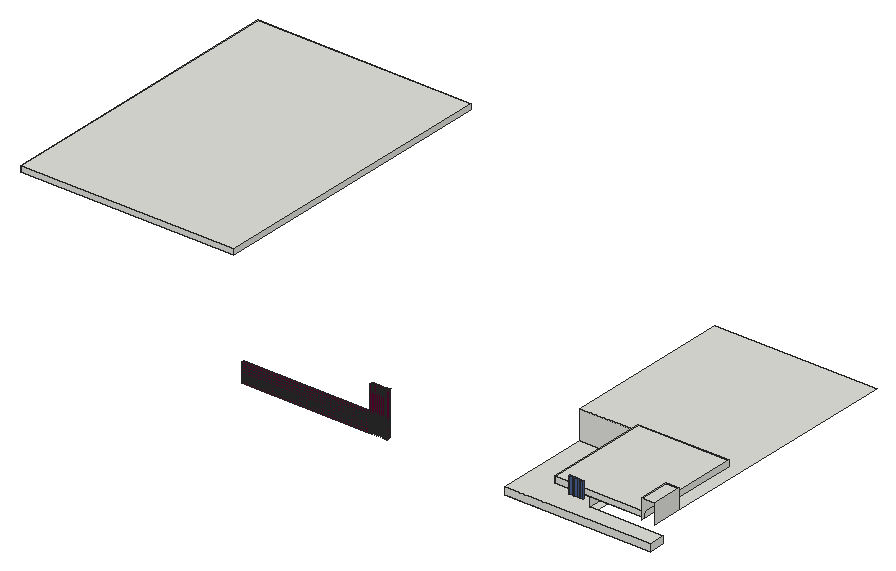
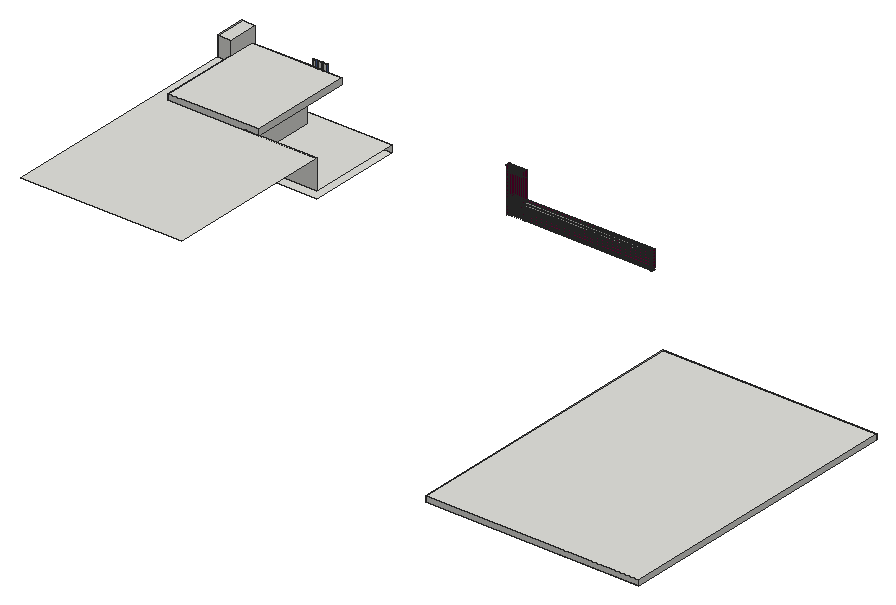
# SketchUp Ruby script. Lengths in inches.
U = 1.inch
M = Sketchup.active_model
def pt(a) = Geom::Point3d.new(a.map { |v| v * U })
def face(e, loops, mat)
  f = e.add_face(loops[0].map { |a| pt(a) })
  loops[1..].each { |l| e.add_face(l.map { |a| pt(a) }).erase! }
  f.material = f.back_material = mat if mat
  f
end
# faces: each face lists its corners as indices into pts; further lists are holes
def faces(e, pts, list, mat = nil) = list.each { |f| face(e, (f[0].is_a?(Array) ? f : [f]).map { |l| l.map { |i| pts[i] } }, mat) }
# xy, xz, yz: faces in a plane at the given z, y or x. An outline is a flat list of corners, or four numbers for a rectangle; further outlines are holes
def ring(l) = l.size == 4 ? [[l[0], l[1]], [l[2], l[1]], [l[2], l[3]], [l[0], l[3]]] : l.each_slice(2).to_a
def flat(e, list, mat, &to3) = list.each { |f| face(e, (f[0].is_a?(Array) ? f : [f]).map { |l| ring(l).map { |u, v| to3.(u, v) } }, mat) }
def xy(e, z, list, mat = nil) = flat(e, list, mat) { |x, y| [x, y, z] }
def xz(e, y, list, mat = nil) = flat(e, list, mat) { |x, z| [x, y, z] }
def yz(e, x, list, mat = nil) = flat(e, list, mat) { |y, z| [x, y, z] }
def lines(e, pts, list) = list.each { |a, b| e.add_line(pt(pts[a]), pt(pts[b])) }
# prism: a flat outline (further loops are holes) pulled along v
def prism(e, loops, v, mat = nil)
  f = face(e, loops, mat); d = Geom::Vector3d.new(v.map { |x| x * U })
  f.pushpull(f.normal.samedirection?(d) ? d.length : -d.length)
end
def box(e, o, s, mat = nil) = prism(e, [[o, [o[0] + s[0], o[1], o[2]], [o[0] + s[0], o[1] + s[1], o[2]], [o[0], o[1] + s[1], o[2]]]], [0, 0, s[2]], mat)
def at(x, y, z, deg = 0) = Geom::Transformation.translation(pt([x, y, z])) * Geom::Transformation.rotation(ORIGIN, Z_AXIS, deg.degrees)
def axes(o, x, y, z) = Geom::Transformation.new([*x, 0, *y, 0, *z, 0, *pt(o).to_a, 1])
def part(name) = M.definitions.add(name)
# library, detail: a bought-in or finely detailed component or shape, given as its bounding box
def library(name, o, s) = part(name).tap { |d| box(d.entities, o, s) }
def detail(e, o, s) = box(e.add_group.entities, o, s)
def put(e, d, t, mat = nil) = e.add_instance(d, t).tap { |i| i.material = mat if mat }
def group(e, t, mat = nil) = e.add_group.tap { |g| g.transformation = t; g.material = mat if mat }.entities
root = M.entities
M.materials.add("[Color L16]").color = [102, 0, 51]
M.materials.add("[Formica Blue]").color = [71, 97, 152]
c1 = part("Recessed downlight \#2")
detail(c1.entities,[0,0,0],[12.875,12.875,1.625])
box(root,[182.534,303.729,246],[321,447,8])
xy(root,218.208,[[671.442,109.729,862.505,112.729]],"[Color L16]")
xy(root,220.302,[[671.442,109.729,862.505,112.729]],"[Color L16]")
xy(root,222,[[1084.247,87.973,1192.934,229.266],[1192.934,87.973,1303.381,111.973]])
xy(root,222.154,[[671.442,109.729,862.505,112.729]],"[Color L16]")
xy(root,224.248,[[671.442,109.729,862.505,112.729]],"[Color L16]")
xy(root,226.101,[[671.442,109.729,862.505,112.729]],"[Color L16]")
xy(root,228.195,[[671.442,109.729,862.505,112.729]],"[Color L16]")
xy(root,230.047,[[671.442,109.729,862.505,112.729]],"[Color L16]")
xy(root,232.141,[[671.442,109.729,862.505,112.729]],"[Color L16]")
xy(root,232.677,[[1084.247,87.973,1303.381,87.973,1303.381,111.973,1192.934,111.973,1192.934,229.266,1084.247,229.266]])
xy(root,233.993,[[671.442,109.729,862.505,112.729]],"[Color L16]")
xy(root,236.087,[[671.442,109.729,862.505,112.729]],"[Color L16]")
xy(root,237.94,[[671.442,109.729,862.505,112.729]],"[Color L16]")
xy(root,240.034,[[671.442,109.729,862.505,112.729]],"[Color L16]")
xy(root,241.886,[[671.442,109.729,862.505,112.729]],"[Color L16]")
xy(root,243.98,[[671.442,109.729,862.505,112.729]],"[Color L16]")
xy(root,245.953,[[671.442,109.729,862.505,112.729]],"[Color L16]")
xy(root,269.993,[[1210.986,69.91,1216.514,71.91]])
xy(root,269.993,[[1195.298,69.91,1200.826,71.91],[1202.736,69.91,1208.264,71.91]],"[Formica Blue]")
xy(root,275.672,[[889.414,108.916,889.428,112.729],[864.033,109.729,864.088,112.729],[867.208,109.729,867.254,112.729],[868.722,109.729,868.782,112.729],[870.382,109.729,870.419,112.729],
  [871.896,109.729,871.948,112.729],[873.556,109.729,873.585,112.729],[875.071,109.729,875.113,112.729],[876.731,109.729,876.751,112.729],[878.245,109.729,878.279,112.729],
  [879.905,109.729,879.917,112.729],[881.419,109.729,881.445,112.729],[883.079,109.729,883.082,112.729],[884.594,109.729,884.611,112.729],[886.248,110.041,886.254,112.729],
  [887.768,110.041,887.831,112.729],[889.414,112.729,889.428,114.354]],"[Color L16]")
xy(root,275.806,[[1171.934,71.91,1171.934,229.266,1192.934,229.266,1192.934,111.973,1307.818,111.973,1307.818,71.91]])
xy(root,276.1875,[[1307.818,111.973,1327.309,111.973,1327.309,482.785,1084.247,482.785,1084.247,229.266,1307.818,229.266]])
xy(root,284.75,[[1171.934,71.91,1307.818,229.266]])
xy(root,284.941,[[889.428,108.916,890.942,114.354],[864.033,109.729,865.547,112.729],[867.208,109.729,868.722,112.729],[870.382,109.729,871.896,112.729],[873.556,109.729,875.071,112.729],
  [876.731,109.729,878.245,112.729],[879.905,109.729,881.419,112.729],[883.079,109.729,884.594,112.729],[886.254,110.041,887.768,112.729]],"[Color L16]")
xy(root,294,[[1210.986,69.91,1216.514,71.91]],"[Formica Blue]")
xy(root,294.25,[[1195.298,69.91,1200.826,71.91],[1202.736,69.91,1208.264,71.91]],"[Formica Blue]")
xz(root,69.91,[[1195.298,269.993,1200.826,294.25],[1202.736,269.993,1208.264,294.25],[1210.986,269.993,1216.514,294]],"[Formica Blue]")
xz(root,71.91,[[1195.298,269.993,1200.826,275.806],[1202.736,269.993,1208.264,275.806],[1210.986,269.993,1216.514,275.806],[1171.934,275.806,1195.298,284.75],[1195.298,275.806,1200.826,284.75],
  [1200.826,275.806,1202.736,284.75],[1202.736,275.806,1208.264,284.75],[1208.264,275.806,1210.986,284.75],[1210.986,275.806,1216.514,284.75],[1216.514,275.806,1307.818,275.806,1307.643,284.75,1216.514,284.75],
  [1307.818,275.806,1307.818,284.75,1307.643,284.75],[1195.298,284.75,1200.826,294.25],[1202.736,284.75,1208.264,294.25],[1210.986,284.75,1216.514,294]])
xz(root,87.973,[[1084.247,222,1303.381,232.677]])
xz(root,109.729,[[671.442,220.302,862.505,222.154],[671.442,224.248,862.505,226.101],[671.442,228.195,862.505,230.047],[671.442,232.141,862.505,233.993],[671.442,236.087,862.505,237.94],
  [671.442,240.034,862.505,241.886],[671.442,243.98,862.505,245.953]],"[Color L16]")
xz(root,111.973,[[1307.818,275.806,1307.248,304.925,1326.739,305.307,1327.309,276.1875,1307.818,276.1875],[1307.818,275.806,1307.818,276.1875,1327.309,276.1875]])
xz(root,112.729,[[671.442,218.208,862.505,218.329],[671.442,218.329,862.505,220.181],[671.442,220.181,862.505,220.302],[671.442,222.154,862.505,222.275],[671.442,222.275,862.505,224.127],
  [671.442,224.127,862.505,224.248],[671.442,226.101,862.505,226.221],[671.442,226.221,862.505,228.074],[671.442,228.074,862.505,228.195],[671.442,230.047,862.505,230.168],
  [671.442,230.168,862.505,232.02],[671.442,232.02,862.505,232.141],[671.442,233.993,862.505,234.114],[671.442,234.114,862.505,235.967],[671.442,235.967,862.505,236.087],
  [671.442,237.94,862.505,238.061],[671.442,238.061,862.505,239.913],[671.442,239.913,862.505,240.034],[671.442,241.886,862.505,242.007],[671.442,242.007,862.505,243.86],
  [671.442,243.86,862.505,243.98],[867.135,275.672,867.208,284.941],[868.722,275.672,868.795,284.941],[870.309,275.672,870.382,284.941],[871.896,275.672,871.969,284.941],
  [873.483,275.672,873.556,284.941],[875.071,275.672,875.143,284.941],[876.658,275.672,876.731,284.941],[878.245,275.672,878.318,284.941],[879.832,275.672,879.905,284.941],
  [881.419,275.672,881.492,284.941],[883.006,275.672,883.079,284.941],[884.594,275.672,884.667,284.941],[886.181,275.672,886.254,284.941]])
xz(root,112.729,[[887.768,275.672,887.841,284.941]],"[Color L16]")
xz(root,229.266,[[1084.247,232.677,1192.934,232.677,1192.934,275.806,1171.934,275.806,1171.934,276.1875,1084.247,276.1875],[1171.934,275.806,1192.934,276.1875],[1171.934,276.1875,1307.818,284.75]])
yz(root,671.442,[[109.729,220.302,112.729,222.154],[109.729,224.248,112.729,226.101],[109.729,228.195,112.729,230.047],[109.729,232.141,112.729,233.993],[109.729,236.087,112.729,237.94],
  [109.729,240.034,112.729,241.886],[109.729,243.98,112.729,245.953]],"[Color L16]")
yz(root,862.505,[[109.729,220.302,112.729,222.154],[109.729,224.248,112.729,226.101],[109.729,228.195,112.729,230.047],[109.729,232.141,112.729,233.993],[109.729,236.087,112.729,237.94],
  [109.729,240.034,112.729,241.886],[109.729,243.98,112.729,245.953]],"[Color L16]")
yz(root,864.033,[[109.729,275.672,112.729,284.941]],"[Color L16]")
yz(root,864.088,[[109.729,218.208,112.729,218.329],[109.729,218.329,112.729,220.181],[109.729,220.181,112.729,220.302],[109.729,220.302,112.729,222.154],[109.729,222.154,112.729,222.275],
  [109.729,222.275,112.729,224.127],[109.729,224.127,112.729,224.248],[109.729,224.248,112.729,226.101],[109.729,226.101,112.729,226.221],[109.729,226.221,112.729,228.074],
  [109.729,228.074,112.729,228.195],[109.729,228.195,112.729,230.047],[109.729,230.047,112.729,230.168],[109.729,230.168,112.729,232.02],[109.729,232.02,112.729,232.141],
  [109.729,232.141,112.729,233.993],[109.729,233.993,112.729,234.114],[109.729,234.114,112.729,235.967],[109.729,235.967,112.729,236.087],[109.729,236.087,112.729,237.94],
  [109.729,237.94,112.729,238.061],[109.729,238.061,112.729,239.913],[109.729,239.913,112.729,240.034],[109.729,240.034,112.729,241.886],[109.729,241.886,112.729,242.007],
  [109.729,242.007,112.729,243.86],[109.729,243.86,112.729,243.98],[109.729,243.98,112.729,245.953],[109.729,245.953,112.729,275.672]],"[Color L16]")
yz(root,867.208,[[109.729,275.672,112.729,284.941]],"[Color L16]")
yz(root,867.254,[[109.729,218.208,112.729,218.329],[109.729,218.329,112.729,220.181],[109.729,220.181,112.729,220.302],[109.729,220.302,112.729,222.154],[109.729,222.154,112.729,222.275],
  [109.729,222.275,112.729,224.127],[109.729,224.127,112.729,224.248],[109.729,224.248,112.729,226.101],[109.729,226.101,112.729,226.221],[109.729,226.221,112.729,228.074],
  [109.729,228.074,112.729,228.195],[109.729,228.195,112.729,230.047],[109.729,230.047,112.729,230.168],[109.729,230.168,112.729,232.02],[109.729,232.02,112.729,232.141],
  [109.729,232.141,112.729,233.993],[109.729,233.993,112.729,234.114],[109.729,234.114,112.729,235.967],[109.729,235.967,112.729,236.087],[109.729,236.087,112.729,237.94],
  [109.729,237.94,112.729,238.061],[109.729,238.061,112.729,239.913],[109.729,239.913,112.729,240.034],[109.729,240.034,112.729,241.886],[109.729,241.886,112.729,242.007],
  [109.729,242.007,112.729,243.86],[109.729,243.86,112.729,243.98],[109.729,243.98,112.729,245.953],[109.729,245.953,112.729,275.672]],"[Color L16]")
yz(root,868.722,[[109.729,275.672,112.729,284.941]],"[Color L16]")
yz(root,870.382,[[109.729,275.672,112.729,284.941]],"[Color L16]")
yz(root,870.419,[[109.729,218.208,112.729,218.329],[109.729,218.329,112.729,220.181],[109.729,220.181,112.729,220.302],[109.729,220.302,112.729,222.154],[109.729,222.154,112.729,222.275],
  [109.729,222.275,112.729,224.127],[109.729,224.127,112.729,224.248],[109.729,224.248,112.729,226.101],[109.729,226.101,112.729,226.221],[109.729,226.221,112.729,228.074],
  [109.729,228.074,112.729,228.195],[109.729,228.195,112.729,230.047],[109.729,230.047,112.729,230.168],[109.729,230.168,112.729,232.02],[109.729,232.02,112.729,232.141],
  [109.729,232.141,112.729,233.993],[109.729,233.993,112.729,234.114],[109.729,234.114,112.729,235.967],[109.729,235.967,112.729,236.087],[109.729,236.087,112.729,237.94],
  [109.729,237.94,112.729,238.061],[109.729,238.061,112.729,239.913],[109.729,239.913,112.729,240.034],[109.729,240.034,112.729,241.886],[109.729,241.886,112.729,242.007],
  [109.729,242.007,112.729,243.86],[109.729,243.86,112.729,243.98],[109.729,243.98,112.729,245.953],[109.729,245.953,112.729,275.672]],"[Color L16]")
yz(root,871.896,[[109.729,275.672,112.729,284.941]],"[Color L16]")
yz(root,873.556,[[109.729,275.672,112.729,284.941]],"[Color L16]")
yz(root,873.585,[[109.729,218.208,112.729,218.329],[109.729,218.329,112.729,220.181],[109.729,220.181,112.729,220.302],[109.729,220.302,112.729,222.154],[109.729,222.154,112.729,222.275],
  [109.729,222.275,112.729,224.127],[109.729,224.127,112.729,224.248],[109.729,224.248,112.729,226.101],[109.729,226.101,112.729,226.221],[109.729,226.221,112.729,228.074],
  [109.729,228.074,112.729,228.195],[109.729,228.195,112.729,230.047],[109.729,230.047,112.729,230.168],[109.729,230.168,112.729,232.02],[109.729,232.02,112.729,232.141],
  [109.729,232.141,112.729,233.993],[109.729,233.993,112.729,234.114],[109.729,234.114,112.729,235.967],[109.729,235.967,112.729,236.087],[109.729,236.087,112.729,237.94],
  [109.729,237.94,112.729,238.061],[109.729,238.061,112.729,239.913],[109.729,239.913,112.729,240.034],[109.729,240.034,112.729,241.886],[109.729,241.886,112.729,242.007],
  [109.729,242.007,112.729,243.86],[109.729,243.86,112.729,243.98],[109.729,243.98,112.729,245.953],[109.729,245.953,112.729,275.672]],"[Color L16]")
yz(root,875.071,[[109.729,275.672,112.729,284.941]],"[Color L16]")
yz(root,876.731,[[109.729,275.672,112.729,284.941]],"[Color L16]")
yz(root,876.751,[[109.729,218.208,112.729,218.329],[109.729,218.329,112.729,220.181],[109.729,220.181,112.729,220.302],[109.729,220.302,112.729,222.154],[109.729,222.154,112.729,222.275],
  [109.729,222.275,112.729,224.127],[109.729,224.127,112.729,224.248],[109.729,224.248,112.729,226.101],[109.729,226.101,112.729,226.221],[109.729,226.221,112.729,228.074],
  [109.729,228.074,112.729,228.195],[109.729,228.195,112.729,230.047],[109.729,230.047,112.729,230.168],[109.729,230.168,112.729,232.02],[109.729,232.02,112.729,232.141],
  [109.729,232.141,112.729,233.993],[109.729,233.993,112.729,234.114],[109.729,234.114,112.729,235.967],[109.729,235.967,112.729,236.087],[109.729,236.087,112.729,237.94],
  [109.729,237.94,112.729,238.061],[109.729,238.061,112.729,239.913],[109.729,239.913,112.729,240.034],[109.729,240.034,112.729,241.886],[109.729,241.886,112.729,242.007],
  [109.729,242.007,112.729,243.86],[109.729,243.86,112.729,243.98],[109.729,243.98,112.729,245.953],[109.729,245.953,112.729,275.672]],"[Color L16]")
yz(root,878.245,[[109.729,275.672,112.729,284.941]],"[Color L16]")
yz(root,879.905,[[109.729,275.672,112.729,284.941]],"[Color L16]")
yz(root,879.917,[[109.729,218.208,112.729,218.329],[109.729,218.329,112.729,220.181],[109.729,220.181,112.729,220.302],[109.729,220.302,112.729,222.154],[109.729,222.154,112.729,222.275],
  [109.729,222.275,112.729,224.127],[109.729,224.127,112.729,224.248],[109.729,224.248,112.729,226.101],[109.729,226.101,112.729,226.221],[109.729,226.221,112.729,228.074],
  [109.729,228.074,112.729,228.195],[109.729,228.195,112.729,230.047],[109.729,230.047,112.729,230.168],[109.729,230.168,112.729,232.02],[109.729,232.02,112.729,232.141],
  [109.729,232.141,112.729,233.993],[109.729,233.993,112.729,234.114],[109.729,234.114,112.729,235.967],[109.729,235.967,112.729,236.087],[109.729,236.087,112.729,237.94],
  [109.729,237.94,112.729,238.061],[109.729,238.061,112.729,239.913],[109.729,239.913,112.729,240.034],[109.729,240.034,112.729,241.886],[109.729,241.886,112.729,242.007],
  [109.729,242.007,112.729,243.86],[109.729,243.86,112.729,243.98],[109.729,243.98,112.729,245.953],[109.729,245.953,112.729,275.672]],"[Color L16]")
yz(root,881.419,[[109.729,275.672,112.729,284.941]],"[Color L16]")
yz(root,883.079,[[109.729,275.672,112.729,284.941]],"[Color L16]")
yz(root,883.082,[[109.729,218.208,112.729,218.329],[109.729,218.329,112.729,220.181],[109.729,220.181,112.729,220.302],[109.729,220.302,112.729,222.154],[109.729,222.154,112.729,222.275],
  [109.729,222.275,112.729,224.127],[109.729,224.127,112.729,224.248],[109.729,224.248,112.729,226.101],[109.729,226.101,112.729,226.221],[109.729,226.221,112.729,228.074],
  [109.729,228.074,112.729,228.195],[109.729,228.195,112.729,230.047],[109.729,230.047,112.729,230.168],[109.729,230.168,112.729,232.02],[109.729,232.02,112.729,232.141],
  [109.729,232.141,112.729,233.993],[109.729,233.993,112.729,234.114],[109.729,234.114,112.729,235.967],[109.729,235.967,112.729,236.087],[109.729,236.087,112.729,237.94],
  [109.729,237.94,112.729,238.061],[109.729,238.061,112.729,239.913],[109.729,239.913,112.729,240.034],[109.729,240.034,112.729,241.886],[109.729,241.886,112.729,242.007],
  [109.729,242.007,112.729,243.86],[109.729,243.86,112.729,243.98],[109.729,243.98,112.729,245.953],[109.729,245.953,112.729,275.672]],"[Color L16]")
yz(root,884.594,[[109.729,275.672,112.729,284.941]],"[Color L16]")
yz(root,886.248,[[110.041,218.208,112.729,218.329],[110.041,218.329,112.729,220.181],[110.041,220.181,112.729,220.302],[110.041,220.302,112.729,222.154],[110.041,222.154,112.729,222.275],
  [110.041,222.275,112.729,224.127],[110.041,224.127,112.729,224.248],[110.041,224.248,112.729,226.101],[110.041,226.101,112.729,226.221],[110.041,226.221,112.729,228.074],
  [110.041,228.074,112.729,228.195],[110.041,228.195,112.729,230.047],[110.041,230.047,112.729,230.168],[110.041,230.168,112.729,232.02],[110.041,232.02,112.729,232.141],
  [110.041,232.141,112.729,233.993],[110.041,233.993,112.729,234.114],[110.041,234.114,112.729,235.967],[110.041,235.967,112.729,236.087],[110.041,236.087,112.729,237.94],
  [110.041,237.94,112.729,238.061],[110.041,238.061,112.729,239.913],[110.041,239.913,112.729,240.034],[110.041,240.034,112.729,241.886],[110.041,241.886,112.729,242.007],
  [110.041,242.007,112.729,243.86],[110.041,243.86,112.729,243.98],[110.041,243.98,112.729,245.953],[110.041,245.953,112.729,275.672]],"[Color L16]")
yz(root,886.254,[[110.041,275.672,112.729,284.941]],"[Color L16]")
yz(root,887.768,[[110.041,275.672,112.729,284.941]],"[Color L16]")
yz(root,887.831,[[110.041,218.208,112.729,218.329],[110.041,218.329,112.729,220.181],[110.041,220.181,112.729,220.302],[110.041,220.302,112.729,222.154],[110.041,222.154,112.729,222.275],
  [110.041,222.275,112.729,224.127],[110.041,224.127,112.729,224.248],[110.041,224.248,112.729,226.101],[110.041,226.101,112.729,226.221],[110.041,226.221,112.729,228.074],
  [110.041,228.074,112.729,228.195],[110.041,228.195,112.729,230.047],[110.041,230.047,112.729,230.168],[110.041,230.168,112.729,232.02],[110.041,232.02,112.729,232.141],
  [110.041,232.141,112.729,233.993],[110.041,233.993,112.729,234.114],[110.041,234.114,112.729,235.967],[110.041,235.967,112.729,236.087],[110.041,236.087,112.729,237.94],
  [110.041,237.94,112.729,238.061],[110.041,238.061,112.729,239.913],[110.041,239.913,112.729,240.034],[110.041,240.034,112.729,241.886],[110.041,241.886,112.729,242.007],
  [110.041,242.007,112.729,243.86],[110.041,243.86,112.729,243.98],[110.041,243.98,112.729,245.953],[110.041,245.953,112.729,275.672]],"[Color L16]")
yz(root,889.414,[[108.916,218.208,112.729,218.329],[112.729,218.208,114.354,218.329],[108.916,218.329,112.729,220.181],[112.729,218.329,114.354,220.181],[108.916,220.181,112.729,220.302],
  [112.729,220.181,114.354,220.302],[108.916,220.302,112.729,222.154],[112.729,220.302,114.354,222.154],[108.916,222.154,112.729,222.275],[112.729,222.154,114.354,222.275],
  [108.916,222.275,112.729,224.127],[112.729,222.275,114.354,224.127],[108.916,224.127,112.729,224.248],[112.729,224.127,114.354,224.248],[108.916,224.248,112.729,226.101],
  [112.729,224.248,114.354,226.101],[108.916,226.101,112.729,226.221],[112.729,226.101,114.354,226.221],[108.916,226.221,112.729,228.074],[112.729,226.221,114.354,228.074],
  [108.916,228.074,112.729,228.195],[112.729,228.074,114.354,228.195],[108.916,228.195,112.729,230.047],[112.729,228.195,114.354,230.047],[108.916,230.047,112.729,230.168],
  [112.729,230.047,114.354,230.168],[108.916,230.168,112.729,232.02],[112.729,230.168,114.354,232.02],[108.916,232.02,112.729,232.141],[112.729,232.02,114.354,232.141],
  [108.916,232.141,112.729,233.993],[112.729,232.141,114.354,233.993],[108.916,233.993,112.729,234.114],[112.729,233.993,114.354,234.114],[108.916,234.114,112.729,235.967],
  [112.729,234.114,114.354,235.967],[108.916,235.967,112.729,236.087],[112.729,235.967,114.354,236.087],[108.916,236.087,112.729,237.94],[112.729,236.087,114.354,237.94],
  [108.916,237.94,112.729,238.061],[112.729,237.94,114.354,238.061],[108.916,238.061,112.729,239.913],[112.729,238.061,114.354,239.913],[108.916,239.913,112.729,240.034],
  [112.729,239.913,114.354,240.034],[108.916,240.034,112.729,241.886],[112.729,240.034,114.354,241.886],[108.916,241.886,112.729,242.007],[112.729,241.886,114.354,242.007],
  [108.916,242.007,112.729,243.86],[112.729,242.007,114.354,243.86],[108.916,243.86,112.729,243.98],[112.729,243.86,114.354,243.98],[108.916,243.98,112.729,245.953],
  [112.729,243.98,114.354,245.953],[108.916,245.953,112.729,275.672],[112.729,245.953,114.354,275.672]],"[Color L16]")
yz(root,889.428,[[108.916,275.672,112.729,284.941],[112.729,275.672,114.354,284.941]],"[Color L16]")
yz(root,1171.934,[[71.91,275.806,229.266,284.75]])
yz(root,1192.934,[[111.973,232.677,229.266,275.806]])
yz(root,1195.298,[[69.91,269.993,71.91,294.25]],"[Formica Blue]")
yz(root,1200.826,[[69.91,269.993,71.91,294.25]],"[Formica Blue]")
yz(root,1202.736,[[69.91,269.993,71.91,294.25]],"[Formica Blue]")
yz(root,1208.264,[[69.91,269.993,71.91,294.25]],"[Formica Blue]")
yz(root,1210.986,[[69.91,269.993,71.91,294]],"[Formica Blue]")
yz(root,1216.514,[[69.91,269.993,71.91,294]],"[Formica Blue]")
yz(root,1303.381,[[87.973,222,111.973,232.677]])
yz(root,1307.818,[[71.91,275.806,111.973,275.806,111.973,276.1875,229.266,276.1875,229.266,284.75,71.91,284.75]])
p = [[1307.818,111.973,275.806],[1307.818,71.91,275.806],[1307.818,65.973,275.806],[1307.248,65.973,304.925],[1307.248,111.973,304.925],[1327.309,65.973,276.1875],
  [1327.309,111.973,276.1875],[1326.739,111.973,305.307],[1326.739,65.973,305.307],[865.671,112.729,243.98],[865.671,112.729,245.953],[865.671,112.729,243.86],
  [865.671,112.729,242.007],[865.671,112.729,241.886],[865.671,112.729,240.034],[865.671,112.729,239.913],[865.671,112.729,238.061],[865.671,112.729,237.94],
  [865.671,112.729,236.087],[865.671,112.729,235.967],[865.671,112.729,234.114],[865.671,112.729,233.993],[865.671,112.729,232.141],[865.671,112.729,232.02],
  [865.671,112.729,230.168],[865.671,112.729,230.047],[865.671,112.729,228.195],[865.671,112.729,228.074],[865.671,112.729,226.221],[865.671,112.729,226.101],
  [865.671,112.729,224.248],[865.671,112.729,224.127],[865.671,112.729,222.275],[865.671,112.729,222.154],[865.671,112.729,220.302],[865.671,112.729,220.181],
  [865.671,112.729,218.329],[865.671,112.729,218.208],[867.262,112.729,275.672],[867.254,112.729,275.672],[868.849,112.729,275.672],[868.836,112.729,275.672],
  [870.436,112.729,275.672],[870.419,112.729,275.672],[872.024,112.729,275.672],[872.002,112.729,275.672],[873.611,112.729,275.672],[873.585,112.729,275.672],
  [875.198,112.729,275.672],[875.168,112.729,275.672],[876.785,112.729,275.672],[876.751,112.729,275.672],[878.372,112.729,275.672],[878.334,112.729,275.672],
  [879.96,112.729,275.672],[879.917,112.729,275.672],[881.547,112.729,275.672],[881.5,112.729,275.672],[883.134,112.729,275.672],[883.082,112.729,275.672],
  [884.721,112.729,275.672],[884.667,112.729,275.672],[886.308,112.729,275.672],[886.254,112.729,275.672],[889.483,112.729,275.672],[889.428,112.729,275.672],
  [1307.818,140.908,275.806]]
faces(root,p,[[0,1,2,3,4],[5,6,7,8],[7,4,3,8]])
lines(root,p,[[9,10],[11,9],[12,11],[13,12],[14,13],[15,14],[16,15],[17,16],[18,17],[19,18],[20,19],[21,20],
  [22,21],[23,22],[24,23],[25,24],[26,25],[27,26],[28,27],[29,28],[30,29],[31,30],[32,31],[33,32],
  [34,33],[35,34],[36,35],[37,36],[38,39],[40,41],[42,43],[44,45],[46,47],[48,49],[50,51],[52,53],
  [54,55],[56,57],[58,59],[60,61],[62,63],[64,65],[0,66]])
put(root,c1,axes([1113.78,162.45,222],[-1,0,0],[0,1,0],[0,0,-1]))
put(root,c1,axes([1159.41,162.45,222],[-1,0,0],[0,1,0],[0,0,-1]))
put(root,c1,axes([1113.78,96.88,222],[-1,0,0],[0,1,0],[0,0,-1]))
put(root,c1,axes([1159.41,108.13,222],[-1,0,0],[0,1,0],[0,0,-1]))
